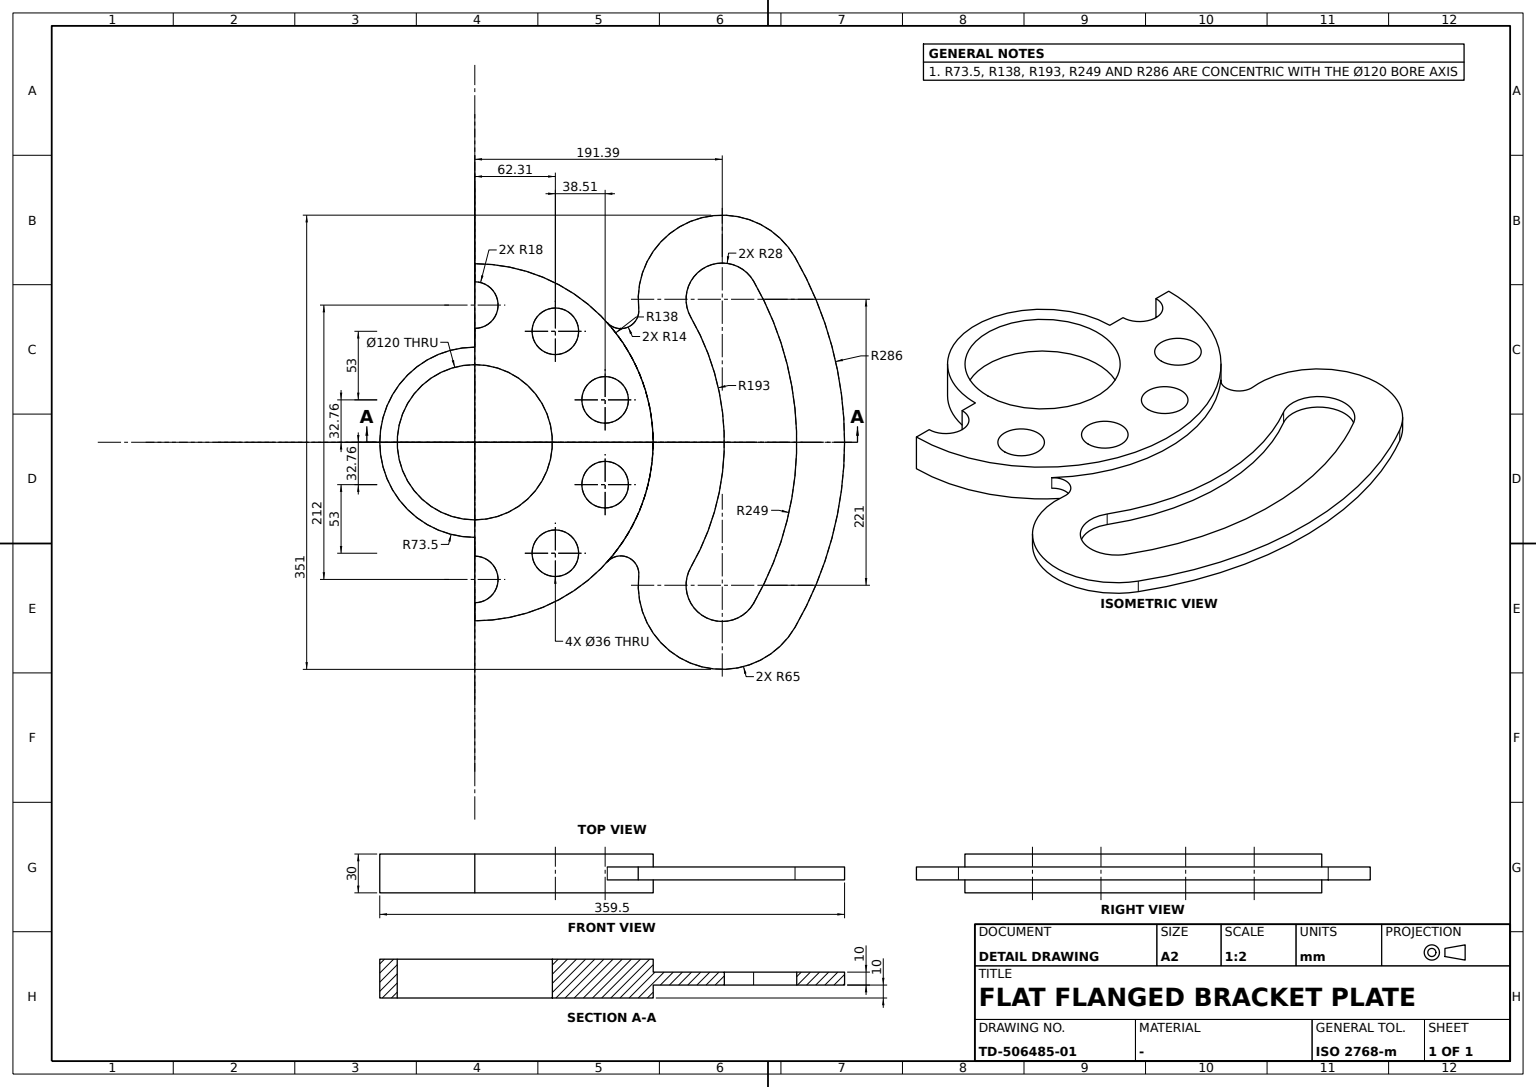
ISO-10303-21;
HEADER;
FILE_DESCRIPTION((''),'2;1');
FILE_NAME('','',(''),(''),'','','');
FILE_SCHEMA(('AUTOMOTIVE_DESIGN'));
ENDSEC;
DATA;
#1=APPLICATION_CONTEXT('');
#2=PRODUCT_CONTEXT('',#1,'mechanical');
#3=PRODUCT('','','',(#2));
#4=PRODUCT_DEFINITION_FORMATION('','',#3);
#5=PRODUCT_DEFINITION_CONTEXT('',#1,'design');
#6=PRODUCT_DEFINITION('','',#4,#5);
#7=PRODUCT_DEFINITION_SHAPE('','',#6);
#8=(LENGTH_UNIT()NAMED_UNIT(*)SI_UNIT(.MILLI.,.METRE.));
#9=(NAMED_UNIT(*)PLANE_ANGLE_UNIT()SI_UNIT($,.RADIAN.));
#10=(NAMED_UNIT(*)SI_UNIT($,.STERADIAN.)SOLID_ANGLE_UNIT());
#11=UNCERTAINTY_MEASURE_WITH_UNIT(LENGTH_MEASURE(0.005),#8,'distance_accuracy_value','');
#12=(GEOMETRIC_REPRESENTATION_CONTEXT(3)GLOBAL_UNCERTAINTY_ASSIGNED_CONTEXT((#11))GLOBAL_UNIT_ASSIGNED_CONTEXT((#8,#9,#10))REPRESENTATION_CONTEXT('',''));
#13=CARTESIAN_POINT('',(-67.7558014,62.3052367,-15.));
#14=VERTEX_POINT('',#13);
#15=CARTESIAN_POINT('',(-85.7558014,62.3052367,-15.));
#16=DIRECTION('',(0.,0.,1.));
#17=DIRECTION('',(1.,0.,0.));
#18=AXIS2_PLACEMENT_3D('',#15,#16,#17);
#19=CIRCLE('',#18,18.);
#20=EDGE_CURVE('',#14,#14,#19,.T.);
#21=ORIENTED_EDGE('',*,*,#20,.F.);
#22=EDGE_LOOP('',(#21));
#23=FACE_BOUND('',#22,.T.);
#24=CARTESIAN_POINT('',(-67.7558014,62.3052367,15.));
#25=VERTEX_POINT('',#24);
#26=CARTESIAN_POINT('',(-85.7558014,62.3052367,15.));
#27=AXIS2_PLACEMENT_3D('',#26,#16,#17);
#28=CIRCLE('',#27,18.);
#29=EDGE_CURVE('',#25,#25,#28,.T.);
#30=ORIENTED_EDGE('',*,*,#29,.T.);
#31=EDGE_LOOP('',(#30));
#32=FACE_BOUND('',#31,.T.);
#33=CARTESIAN_POINT('',(-85.7558014,62.3052367,0.));
#34=DIRECTION('',(-0.809016994,0.587785252,0.));
#35=AXIS2_PLACEMENT_3D('',#33,#16,#34);
#36=CYLINDRICAL_SURFACE('',#35,18.);
#37=ADVANCED_FACE('',(#23,#32),#36,.F.);
#38=CARTESIAN_POINT('',(96.5,167.1429029,5.));
#39=VERTEX_POINT('',#38);
#40=CARTESIAN_POINT('',(-96.5,167.1429029,5.));
#41=VERTEX_POINT('',#40);
#42=CARTESIAN_POINT('',(0.,0.,5.));
#43=AXIS2_PLACEMENT_3D('',#42,#16,#17);
#44=CIRCLE('',#43,193.);
#45=EDGE_CURVE('',#39,#41,#44,.T.);
#46=ORIENTED_EDGE('',*,*,#45,.F.);
#47=CARTESIAN_POINT('',(96.5,167.1429029,-5.));
#48=VERTEX_POINT('',#47);
#49=CARTESIAN_POINT('',(96.5,167.1429029,0.));
#50=VECTOR('',#16,1000.);
#51=LINE('',#49,#50);
#52=EDGE_CURVE('',#48,#39,#51,.T.);
#53=ORIENTED_EDGE('',*,*,#52,.F.);
#54=CARTESIAN_POINT('',(-96.5,167.1429029,-5.));
#55=VERTEX_POINT('',#54);
#56=CARTESIAN_POINT('',(0.,0.,-5.));
#57=AXIS2_PLACEMENT_3D('',#56,#16,#17);
#58=CIRCLE('',#57,193.);
#59=EDGE_CURVE('',#48,#55,#58,.T.);
#60=ORIENTED_EDGE('',*,*,#59,.T.);
#61=CARTESIAN_POINT('',(-96.5,167.1429029,0.));
#62=LINE('',#61,#50);
#63=EDGE_CURVE('',#55,#41,#62,.T.);
#64=ORIENTED_EDGE('',*,*,#63,.T.);
#65=EDGE_LOOP('',(#46,#53,#60,#64));
#66=FACE_BOUND('',#65,.T.);
#67=CARTESIAN_POINT('',(0.,0.,0.));
#68=AXIS2_PLACEMENT_3D('',#67,#16,#17);
#69=CYLINDRICAL_SURFACE('',#68,193.);
#70=ADVANCED_FACE('',(#66),#69,.T.);
#71=CARTESIAN_POINT('',(73.5,0.,-15.));
#72=VERTEX_POINT('',#71);
#73=CARTESIAN_POINT('',(88.,0.,-15.));
#74=VERTEX_POINT('',#73);
#75=CARTESIAN_POINT('',(-73.5,0.,-15.));
#76=VECTOR('',#17,1000.);
#77=LINE('',#75,#76);
#78=EDGE_CURVE('',#72,#74,#77,.T.);
#79=ORIENTED_EDGE('',*,*,#78,.T.);
#80=CARTESIAN_POINT('',(88.,0.,15.));
#81=VERTEX_POINT('',#80);
#82=LINE('',#73,#50);
#83=EDGE_CURVE('',#81,#74,#82,.F.);
#84=ORIENTED_EDGE('',*,*,#83,.F.);
#85=CARTESIAN_POINT('',(73.5,0.,15.));
#86=VERTEX_POINT('',#85);
#87=CARTESIAN_POINT('',(-73.5,0.,15.));
#88=LINE('',#87,#76);
#89=EDGE_CURVE('',#86,#81,#88,.T.);
#90=ORIENTED_EDGE('',*,*,#89,.F.);
#91=LINE('',#71,#50);
#92=EDGE_CURVE('',#72,#86,#91,.T.);
#93=ORIENTED_EDGE('',*,*,#92,.F.);
#94=EDGE_LOOP('',(#79,#84,#90,#93));
#95=FACE_BOUND('',#94,.T.);
#96=CARTESIAN_POINT('',(-73.5,0.,0.));
#97=DIRECTION('',(0.,1.,0.));
#98=DIRECTION('',(-1.,0.,0.));
#99=AXIS2_PLACEMENT_3D('',#96,#97,#98);
#100=PLANE('',#99);
#101=ADVANCED_FACE('',(#95),#100,.F.);
#102=CARTESIAN_POINT('',(-14.7558014,100.8119907,-15.));
#103=VERTEX_POINT('',#102);
#104=CARTESIAN_POINT('',(-32.7558014,100.8119907,-15.));
#105=AXIS2_PLACEMENT_3D('',#104,#16,#17);
#106=CIRCLE('',#105,18.);
#107=EDGE_CURVE('',#103,#103,#106,.T.);
#108=ORIENTED_EDGE('',*,*,#107,.F.);
#109=EDGE_LOOP('',(#108));
#110=FACE_BOUND('',#109,.T.);
#111=CARTESIAN_POINT('',(-14.7558014,100.8119907,15.));
#112=VERTEX_POINT('',#111);
#113=CARTESIAN_POINT('',(-32.7558014,100.8119907,15.));
#114=AXIS2_PLACEMENT_3D('',#113,#16,#17);
#115=CIRCLE('',#114,18.);
#116=EDGE_CURVE('',#112,#112,#115,.T.);
#117=ORIENTED_EDGE('',*,*,#116,.T.);
#118=EDGE_LOOP('',(#117));
#119=FACE_BOUND('',#118,.T.);
#120=CARTESIAN_POINT('',(-32.7558014,100.8119907,0.));
#121=DIRECTION('',(-0.309016994,0.951056516,0.));
#122=AXIS2_PLACEMENT_3D('',#120,#16,#121);
#123=CYLINDRICAL_SURFACE('',#122,18.);
#124=ADVANCED_FACE('',(#110,#119),#123,.F.);
#125=CARTESIAN_POINT('',(124.5,215.6403255,-5.));
#126=VERTEX_POINT('',#125);
#127=CARTESIAN_POINT('',(110.5,191.3916142,-5.));
#128=AXIS2_PLACEMENT_3D('',#127,#16,#17);
#129=CIRCLE('',#128,28.);
#130=EDGE_CURVE('',#48,#126,#129,.T.);
#131=ORIENTED_EDGE('',*,*,#130,.T.);
#132=CARTESIAN_POINT('',(-124.5,215.6403255,-5.));
#133=VERTEX_POINT('',#132);
#134=CIRCLE('',#57,249.);
#135=EDGE_CURVE('',#126,#133,#134,.T.);
#136=ORIENTED_EDGE('',*,*,#135,.T.);
#137=CARTESIAN_POINT('',(-110.5,191.3916142,-5.));
#138=AXIS2_PLACEMENT_3D('',#137,#16,#17);
#139=CIRCLE('',#138,28.);
#140=EDGE_CURVE('',#133,#55,#139,.T.);
#141=ORIENTED_EDGE('',*,*,#140,.T.);
#142=ORIENTED_EDGE('',*,*,#59,.F.);
#143=EDGE_LOOP('',(#131,#136,#141,#142));
#144=FACE_BOUND('',#143,.T.);
#145=CARTESIAN_POINT('',(-92.4269535,102.4756472,-5.));
#146=VERTEX_POINT('',#145);
#147=CARTESIAN_POINT('',(-103.344735,126.786644,-5.));
#148=VERTEX_POINT('',#147);
#149=CARTESIAN_POINT('',(-101.803601,112.8717273,-5.));
#150=AXIS2_PLACEMENT_3D('',#149,#16,#17);
#151=CIRCLE('',#150,14.);
#152=EDGE_CURVE('',#146,#148,#151,.T.);
#153=ORIENTED_EDGE('',*,*,#152,.T.);
#154=CARTESIAN_POINT('',(-143.,247.6832655,-5.));
#155=VERTEX_POINT('',#154);
#156=CIRCLE('',#138,65.);
#157=EDGE_CURVE('',#155,#148,#156,.T.);
#158=ORIENTED_EDGE('',*,*,#157,.F.);
#159=CARTESIAN_POINT('',(143.,247.6832655,-5.));
#160=VERTEX_POINT('',#159);
#161=CIRCLE('',#57,286.);
#162=EDGE_CURVE('',#160,#155,#161,.T.);
#163=ORIENTED_EDGE('',*,*,#162,.F.);
#164=CARTESIAN_POINT('',(103.344735,126.786644,-5.));
#165=VERTEX_POINT('',#164);
#166=CIRCLE('',#128,65.);
#167=EDGE_CURVE('',#165,#160,#166,.T.);
#168=ORIENTED_EDGE('',*,*,#167,.F.);
#169=CARTESIAN_POINT('',(92.4269535,102.4756472,-5.));
#170=VERTEX_POINT('',#169);
#171=CARTESIAN_POINT('',(101.803601,112.8717273,-5.));
#172=AXIS2_PLACEMENT_3D('',#171,#16,#17);
#173=CIRCLE('',#172,14.);
#174=EDGE_CURVE('',#165,#170,#173,.T.);
#175=ORIENTED_EDGE('',*,*,#174,.T.);
#176=CIRCLE('',#57,138.);
#177=EDGE_CURVE('',#170,#146,#176,.T.);
#178=ORIENTED_EDGE('',*,*,#177,.T.);
#179=EDGE_LOOP('',(#153,#158,#163,#168,#175,#178));
#180=FACE_BOUND('',#179,.T.);
#181=PLANE('',#57);
#182=ADVANCED_FACE('',(#144,#180),#181,.F.);
#183=CARTESIAN_POINT('',(60.,0.,15.));
#184=VERTEX_POINT('',#183);
#185=CARTESIAN_POINT('',(0.,0.,15.));
#186=AXIS2_PLACEMENT_3D('',#185,#16,#17);
#187=CIRCLE('',#186,60.);
#188=EDGE_CURVE('',#184,#184,#187,.T.);
#189=ORIENTED_EDGE('',*,*,#188,.T.);
#190=EDGE_LOOP('',(#189));
#191=FACE_BOUND('',#190,.T.);
#192=CARTESIAN_POINT('',(60.,0.,-15.));
#193=VERTEX_POINT('',#192);
#194=CARTESIAN_POINT('',(0.,0.,-15.));
#195=AXIS2_PLACEMENT_3D('',#194,#16,#17);
#196=CIRCLE('',#195,60.);
#197=EDGE_CURVE('',#193,#193,#196,.T.);
#198=ORIENTED_EDGE('',*,*,#197,.F.);
#199=EDGE_LOOP('',(#198));
#200=FACE_BOUND('',#199,.T.);
#201=CYLINDRICAL_SURFACE('',#68,60.);
#202=ADVANCED_FACE('',(#191,#200),#201,.F.);
#203=CARTESIAN_POINT('',(103.7558014,62.3052367,15.));
#204=VERTEX_POINT('',#203);
#205=CARTESIAN_POINT('',(85.7558014,62.3052367,15.));
#206=AXIS2_PLACEMENT_3D('',#205,#16,#17);
#207=CIRCLE('',#206,18.);
#208=EDGE_CURVE('',#204,#204,#207,.T.);
#209=ORIENTED_EDGE('',*,*,#208,.T.);
#210=EDGE_LOOP('',(#209));
#211=FACE_BOUND('',#210,.T.);
#212=CARTESIAN_POINT('',(103.7558014,62.3052367,-15.));
#213=VERTEX_POINT('',#212);
#214=CARTESIAN_POINT('',(85.7558014,62.3052367,-15.));
#215=AXIS2_PLACEMENT_3D('',#214,#16,#17);
#216=CIRCLE('',#215,18.);
#217=EDGE_CURVE('',#213,#213,#216,.T.);
#218=ORIENTED_EDGE('',*,*,#217,.F.);
#219=EDGE_LOOP('',(#218));
#220=FACE_BOUND('',#219,.T.);
#221=CARTESIAN_POINT('',(85.7558014,62.3052367,0.));
#222=DIRECTION('',(0.809016994,0.587785252,0.));
#223=AXIS2_PLACEMENT_3D('',#221,#16,#222);
#224=CYLINDRICAL_SURFACE('',#223,18.);
#225=ADVANCED_FACE('',(#211,#220),#224,.F.);
#226=CARTESIAN_POINT('',(-88.,0.,15.));
#227=VERTEX_POINT('',#226);
#228=CARTESIAN_POINT('',(-124.,0.,15.));
#229=VERTEX_POINT('',#228);
#230=CARTESIAN_POINT('',(-106.,0.,15.));
#231=AXIS2_PLACEMENT_3D('',#230,#16,#17);
#232=CIRCLE('',#231,18.);
#233=EDGE_CURVE('',#227,#229,#232,.T.);
#234=ORIENTED_EDGE('',*,*,#233,.T.);
#235=CARTESIAN_POINT('',(-124.,0.,-15.));
#236=VERTEX_POINT('',#235);
#237=LINE('',#235,#50);
#238=EDGE_CURVE('',#236,#229,#237,.T.);
#239=ORIENTED_EDGE('',*,*,#238,.F.);
#240=CARTESIAN_POINT('',(-88.,0.,-15.));
#241=VERTEX_POINT('',#240);
#242=CARTESIAN_POINT('',(-106.,0.,-15.));
#243=AXIS2_PLACEMENT_3D('',#242,#16,#17);
#244=CIRCLE('',#243,18.);
#245=EDGE_CURVE('',#241,#236,#244,.T.);
#246=ORIENTED_EDGE('',*,*,#245,.F.);
#247=LINE('',#240,#50);
#248=EDGE_CURVE('',#227,#241,#247,.F.);
#249=ORIENTED_EDGE('',*,*,#248,.F.);
#250=EDGE_LOOP('',(#234,#239,#246,#249));
#251=FACE_BOUND('',#250,.T.);
#252=CARTESIAN_POINT('',(-106.,0.,0.));
#253=AXIS2_PLACEMENT_3D('',#252,#16,#98);
#254=CYLINDRICAL_SURFACE('',#253,18.);
#255=ADVANCED_FACE('',(#251),#254,.F.);
#256=CARTESIAN_POINT('',(138.,0.,-15.));
#257=VERTEX_POINT('',#256);
#258=CARTESIAN_POINT('',(138.,0.,15.));
#259=VERTEX_POINT('',#258);
#260=LINE('',#256,#50);
#261=EDGE_CURVE('',#257,#259,#260,.T.);
#262=ORIENTED_EDGE('',*,*,#261,.F.);
#263=CARTESIAN_POINT('',(-138.,0.,-15.));
#264=VERTEX_POINT('',#263);
#265=CIRCLE('',#195,138.);
#266=EDGE_CURVE('',#257,#264,#265,.T.);
#267=ORIENTED_EDGE('',*,*,#266,.T.);
#268=CARTESIAN_POINT('',(-138.,0.,15.));
#269=VERTEX_POINT('',#268);
#270=LINE('',#263,#50);
#271=EDGE_CURVE('',#264,#269,#270,.T.);
#272=ORIENTED_EDGE('',*,*,#271,.T.);
#273=CIRCLE('',#186,138.);
#274=EDGE_CURVE('',#259,#269,#273,.T.);
#275=ORIENTED_EDGE('',*,*,#274,.F.);
#276=EDGE_LOOP('',(#262,#267,#272,#275));
#277=FACE_BOUND('',#276,.T.);
#278=ORIENTED_EDGE('',*,*,#177,.F.);
#279=CARTESIAN_POINT('',(92.4269535,102.4756472,5.));
#280=VERTEX_POINT('',#279);
#281=CARTESIAN_POINT('',(92.4269535,102.4756472,0.));
#282=LINE('',#281,#50);
#283=EDGE_CURVE('',#170,#280,#282,.T.);
#284=ORIENTED_EDGE('',*,*,#283,.T.);
#285=CARTESIAN_POINT('',(-92.4269535,102.4756472,5.));
#286=VERTEX_POINT('',#285);
#287=CIRCLE('',#43,138.);
#288=EDGE_CURVE('',#280,#286,#287,.T.);
#289=ORIENTED_EDGE('',*,*,#288,.T.);
#290=CARTESIAN_POINT('',(-92.4269535,102.4756472,0.));
#291=LINE('',#290,#50);
#292=EDGE_CURVE('',#146,#286,#291,.T.);
#293=ORIENTED_EDGE('',*,*,#292,.F.);
#294=EDGE_LOOP('',(#278,#284,#289,#293));
#295=FACE_BOUND('',#294,.T.);
#296=CYLINDRICAL_SURFACE('',#68,138.);
#297=ADVANCED_FACE('',(#277,#295),#296,.T.);
#298=ORIENTED_EDGE('',*,*,#63,.F.);
#299=ORIENTED_EDGE('',*,*,#140,.F.);
#300=CARTESIAN_POINT('',(-124.5,215.6403255,5.));
#301=VERTEX_POINT('',#300);
#302=CARTESIAN_POINT('',(-124.5,215.6403255,0.));
#303=LINE('',#302,#50);
#304=EDGE_CURVE('',#133,#301,#303,.T.);
#305=ORIENTED_EDGE('',*,*,#304,.T.);
#306=CARTESIAN_POINT('',(-110.5,191.3916142,5.));
#307=AXIS2_PLACEMENT_3D('',#306,#16,#17);
#308=CIRCLE('',#307,28.);
#309=EDGE_CURVE('',#301,#41,#308,.T.);
#310=ORIENTED_EDGE('',*,*,#309,.T.);
#311=EDGE_LOOP('',(#298,#299,#305,#310));
#312=FACE_BOUND('',#311,.T.);
#313=CARTESIAN_POINT('',(-110.5,191.3916142,0.));
#314=AXIS2_PLACEMENT_3D('',#313,#16,#17);
#315=CYLINDRICAL_SURFACE('',#314,28.);
#316=ADVANCED_FACE('',(#312),#315,.F.);
#317=ORIENTED_EDGE('',*,*,#238,.T.);
#318=EDGE_CURVE('',#269,#229,#88,.T.);
#319=ORIENTED_EDGE('',*,*,#318,.F.);
#320=ORIENTED_EDGE('',*,*,#271,.F.);
#321=EDGE_CURVE('',#264,#236,#77,.T.);
#322=ORIENTED_EDGE('',*,*,#321,.T.);
#323=EDGE_LOOP('',(#317,#319,#320,#322));
#324=FACE_BOUND('',#323,.T.);
#325=ADVANCED_FACE('',(#324),#100,.F.);
#326=CARTESIAN_POINT('',(50.7558014,100.8119907,-15.));
#327=VERTEX_POINT('',#326);
#328=CARTESIAN_POINT('',(32.7558014,100.8119907,-15.));
#329=AXIS2_PLACEMENT_3D('',#328,#16,#17);
#330=CIRCLE('',#329,18.);
#331=EDGE_CURVE('',#327,#327,#330,.T.);
#332=ORIENTED_EDGE('',*,*,#331,.F.);
#333=EDGE_LOOP('',(#332));
#334=FACE_BOUND('',#333,.T.);
#335=CARTESIAN_POINT('',(50.7558014,100.8119907,15.));
#336=VERTEX_POINT('',#335);
#337=CARTESIAN_POINT('',(32.7558014,100.8119907,15.));
#338=AXIS2_PLACEMENT_3D('',#337,#16,#17);
#339=CIRCLE('',#338,18.);
#340=EDGE_CURVE('',#336,#336,#339,.T.);
#341=ORIENTED_EDGE('',*,*,#340,.T.);
#342=EDGE_LOOP('',(#341));
#343=FACE_BOUND('',#342,.T.);
#344=CARTESIAN_POINT('',(32.7558014,100.8119907,0.));
#345=DIRECTION('',(0.309016994,0.951056516,0.));
#346=AXIS2_PLACEMENT_3D('',#344,#16,#345);
#347=CYLINDRICAL_SURFACE('',#346,18.);
#348=ADVANCED_FACE('',(#334,#343),#347,.F.);
#349=ORIENTED_EDGE('',*,*,#340,.F.);
#350=EDGE_LOOP('',(#349));
#351=FACE_BOUND('',#350,.T.);
#352=CARTESIAN_POINT('',(124.,0.,15.));
#353=VERTEX_POINT('',#352);
#354=CARTESIAN_POINT('',(106.,0.,15.));
#355=AXIS2_PLACEMENT_3D('',#354,#16,#17);
#356=CIRCLE('',#355,18.);
#357=EDGE_CURVE('',#353,#81,#356,.T.);
#358=ORIENTED_EDGE('',*,*,#357,.F.);
#359=EDGE_CURVE('',#353,#259,#88,.T.);
#360=ORIENTED_EDGE('',*,*,#359,.T.);
#361=ORIENTED_EDGE('',*,*,#274,.T.);
#362=ORIENTED_EDGE('',*,*,#318,.T.);
#363=ORIENTED_EDGE('',*,*,#233,.F.);
#364=VERTEX_POINT('',#87);
#365=EDGE_CURVE('',#227,#364,#88,.T.);
#366=ORIENTED_EDGE('',*,*,#365,.T.);
#367=CIRCLE('',#186,73.5);
#368=EDGE_CURVE('',#364,#86,#367,.T.);
#369=ORIENTED_EDGE('',*,*,#368,.T.);
#370=ORIENTED_EDGE('',*,*,#89,.T.);
#371=EDGE_LOOP('',(#358,#360,#361,#362,#363,#366,#369,#370));
#372=FACE_BOUND('',#371,.T.);
#373=ORIENTED_EDGE('',*,*,#188,.F.);
#374=EDGE_LOOP('',(#373));
#375=FACE_BOUND('',#374,.T.);
#376=ORIENTED_EDGE('',*,*,#208,.F.);
#377=EDGE_LOOP('',(#376));
#378=FACE_BOUND('',#377,.T.);
#379=ORIENTED_EDGE('',*,*,#116,.F.);
#380=EDGE_LOOP('',(#379));
#381=FACE_BOUND('',#380,.T.);
#382=ORIENTED_EDGE('',*,*,#29,.F.);
#383=EDGE_LOOP('',(#382));
#384=FACE_BOUND('',#383,.T.);
#385=PLANE('',#186);
#386=ADVANCED_FACE('',(#351,#372,#375,#378,#381,#384),#385,.T.);
#387=CARTESIAN_POINT('',(103.344735,126.786644,5.));
#388=VERTEX_POINT('',#387);
#389=CARTESIAN_POINT('',(101.803601,112.8717273,5.));
#390=AXIS2_PLACEMENT_3D('',#389,#16,#17);
#391=CIRCLE('',#390,14.);
#392=EDGE_CURVE('',#388,#280,#391,.T.);
#393=ORIENTED_EDGE('',*,*,#392,.T.);
#394=ORIENTED_EDGE('',*,*,#283,.F.);
#395=ORIENTED_EDGE('',*,*,#174,.F.);
#396=CARTESIAN_POINT('',(103.344735,126.786644,0.));
#397=LINE('',#396,#50);
#398=EDGE_CURVE('',#165,#388,#397,.T.);
#399=ORIENTED_EDGE('',*,*,#398,.T.);
#400=EDGE_LOOP('',(#393,#394,#395,#399));
#401=FACE_BOUND('',#400,.T.);
#402=CARTESIAN_POINT('',(101.803601,112.8717273,0.));
#403=AXIS2_PLACEMENT_3D('',#402,#16,#17);
#404=CYLINDRICAL_SURFACE('',#403,14.);
#405=ADVANCED_FACE('',(#401),#404,.F.);
#406=CARTESIAN_POINT('',(-103.344735,126.786644,5.));
#407=VERTEX_POINT('',#406);
#408=CARTESIAN_POINT('',(-101.803601,112.8717273,5.));
#409=AXIS2_PLACEMENT_3D('',#408,#16,#17);
#410=CIRCLE('',#409,14.);
#411=EDGE_CURVE('',#286,#407,#410,.T.);
#412=ORIENTED_EDGE('',*,*,#411,.T.);
#413=CARTESIAN_POINT('',(-103.344735,126.786644,0.));
#414=LINE('',#413,#50);
#415=EDGE_CURVE('',#148,#407,#414,.T.);
#416=ORIENTED_EDGE('',*,*,#415,.F.);
#417=ORIENTED_EDGE('',*,*,#152,.F.);
#418=ORIENTED_EDGE('',*,*,#292,.T.);
#419=EDGE_LOOP('',(#412,#416,#417,#418));
#420=FACE_BOUND('',#419,.T.);
#421=CARTESIAN_POINT('',(-101.803601,112.8717273,0.));
#422=AXIS2_PLACEMENT_3D('',#421,#16,#17);
#423=CYLINDRICAL_SURFACE('',#422,14.);
#424=ADVANCED_FACE('',(#420),#423,.F.);
#425=ORIENTED_EDGE('',*,*,#107,.T.);
#426=EDGE_LOOP('',(#425));
#427=FACE_BOUND('',#426,.T.);
#428=ORIENTED_EDGE('',*,*,#331,.T.);
#429=EDGE_LOOP('',(#428));
#430=FACE_BOUND('',#429,.T.);
#431=ORIENTED_EDGE('',*,*,#217,.T.);
#432=EDGE_LOOP('',(#431));
#433=FACE_BOUND('',#432,.T.);
#434=CARTESIAN_POINT('',(124.,0.,-15.));
#435=VERTEX_POINT('',#434);
#436=CARTESIAN_POINT('',(106.,0.,-15.));
#437=AXIS2_PLACEMENT_3D('',#436,#16,#17);
#438=CIRCLE('',#437,18.);
#439=EDGE_CURVE('',#435,#74,#438,.T.);
#440=ORIENTED_EDGE('',*,*,#439,.T.);
#441=ORIENTED_EDGE('',*,*,#78,.F.);
#442=VERTEX_POINT('',#75);
#443=CIRCLE('',#195,73.5);
#444=EDGE_CURVE('',#442,#72,#443,.T.);
#445=ORIENTED_EDGE('',*,*,#444,.F.);
#446=EDGE_CURVE('',#241,#442,#77,.T.);
#447=ORIENTED_EDGE('',*,*,#446,.F.);
#448=ORIENTED_EDGE('',*,*,#245,.T.);
#449=ORIENTED_EDGE('',*,*,#321,.F.);
#450=ORIENTED_EDGE('',*,*,#266,.F.);
#451=EDGE_CURVE('',#435,#257,#77,.T.);
#452=ORIENTED_EDGE('',*,*,#451,.F.);
#453=EDGE_LOOP('',(#440,#441,#445,#447,#448,#449,#450,#452));
#454=FACE_BOUND('',#453,.T.);
#455=ORIENTED_EDGE('',*,*,#20,.T.);
#456=EDGE_LOOP('',(#455));
#457=FACE_BOUND('',#456,.T.);
#458=ORIENTED_EDGE('',*,*,#197,.T.);
#459=EDGE_LOOP('',(#458));
#460=FACE_BOUND('',#459,.T.);
#461=PLANE('',#195);
#462=ADVANCED_FACE('',(#427,#430,#433,#454,#457,#460),#461,.F.);
#463=CARTESIAN_POINT('',(-143.,247.6832655,5.));
#464=VERTEX_POINT('',#463);
#465=CIRCLE('',#307,65.);
#466=EDGE_CURVE('',#464,#407,#465,.T.);
#467=ORIENTED_EDGE('',*,*,#466,.F.);
#468=CARTESIAN_POINT('',(-143.,247.6832655,0.));
#469=LINE('',#468,#50);
#470=EDGE_CURVE('',#155,#464,#469,.T.);
#471=ORIENTED_EDGE('',*,*,#470,.F.);
#472=ORIENTED_EDGE('',*,*,#157,.T.);
#473=ORIENTED_EDGE('',*,*,#415,.T.);
#474=EDGE_LOOP('',(#467,#471,#472,#473));
#475=FACE_BOUND('',#474,.T.);
#476=CYLINDRICAL_SURFACE('',#314,65.);
#477=ADVANCED_FACE('',(#475),#476,.T.);
#478=CARTESIAN_POINT('',(143.,247.6832655,5.));
#479=VERTEX_POINT('',#478);
#480=CIRCLE('',#43,286.);
#481=EDGE_CURVE('',#479,#464,#480,.T.);
#482=ORIENTED_EDGE('',*,*,#481,.F.);
#483=CARTESIAN_POINT('',(143.,247.6832655,0.));
#484=LINE('',#483,#50);
#485=EDGE_CURVE('',#160,#479,#484,.T.);
#486=ORIENTED_EDGE('',*,*,#485,.F.);
#487=ORIENTED_EDGE('',*,*,#162,.T.);
#488=ORIENTED_EDGE('',*,*,#470,.T.);
#489=EDGE_LOOP('',(#482,#486,#487,#488));
#490=FACE_BOUND('',#489,.T.);
#491=CYLINDRICAL_SURFACE('',#68,286.);
#492=ADVANCED_FACE('',(#490),#491,.T.);
#493=ORIENTED_EDGE('',*,*,#446,.T.);
#494=LINE('',#75,#50);
#495=EDGE_CURVE('',#442,#364,#494,.T.);
#496=ORIENTED_EDGE('',*,*,#495,.T.);
#497=ORIENTED_EDGE('',*,*,#365,.F.);
#498=ORIENTED_EDGE('',*,*,#248,.T.);
#499=EDGE_LOOP('',(#493,#496,#497,#498));
#500=FACE_BOUND('',#499,.T.);
#501=ADVANCED_FACE('',(#500),#100,.F.);
#502=ORIENTED_EDGE('',*,*,#167,.T.);
#503=ORIENTED_EDGE('',*,*,#485,.T.);
#504=CARTESIAN_POINT('',(110.5,191.3916142,5.));
#505=AXIS2_PLACEMENT_3D('',#504,#16,#17);
#506=CIRCLE('',#505,65.);
#507=EDGE_CURVE('',#388,#479,#506,.T.);
#508=ORIENTED_EDGE('',*,*,#507,.F.);
#509=ORIENTED_EDGE('',*,*,#398,.F.);
#510=EDGE_LOOP('',(#502,#503,#508,#509));
#511=FACE_BOUND('',#510,.T.);
#512=CARTESIAN_POINT('',(110.5,191.3916142,0.));
#513=AXIS2_PLACEMENT_3D('',#512,#16,#17);
#514=CYLINDRICAL_SURFACE('',#513,65.);
#515=ADVANCED_FACE('',(#511),#514,.T.);
#516=CARTESIAN_POINT('',(124.5,215.6403255,5.));
#517=VERTEX_POINT('',#516);
#518=CARTESIAN_POINT('',(124.5,215.6403255,0.));
#519=LINE('',#518,#50);
#520=EDGE_CURVE('',#126,#517,#519,.T.);
#521=ORIENTED_EDGE('',*,*,#520,.F.);
#522=ORIENTED_EDGE('',*,*,#130,.F.);
#523=ORIENTED_EDGE('',*,*,#52,.T.);
#524=CIRCLE('',#505,28.);
#525=EDGE_CURVE('',#39,#517,#524,.T.);
#526=ORIENTED_EDGE('',*,*,#525,.T.);
#527=EDGE_LOOP('',(#521,#522,#523,#526));
#528=FACE_BOUND('',#527,.T.);
#529=CYLINDRICAL_SURFACE('',#513,28.);
#530=ADVANCED_FACE('',(#528),#529,.F.);
#531=ORIENTED_EDGE('',*,*,#135,.F.);
#532=ORIENTED_EDGE('',*,*,#520,.T.);
#533=CIRCLE('',#43,249.);
#534=EDGE_CURVE('',#517,#301,#533,.T.);
#535=ORIENTED_EDGE('',*,*,#534,.T.);
#536=ORIENTED_EDGE('',*,*,#304,.F.);
#537=EDGE_LOOP('',(#531,#532,#535,#536));
#538=FACE_BOUND('',#537,.T.);
#539=CYLINDRICAL_SURFACE('',#68,249.);
#540=ADVANCED_FACE('',(#538),#539,.F.);
#541=ORIENTED_EDGE('',*,*,#534,.F.);
#542=ORIENTED_EDGE('',*,*,#525,.F.);
#543=ORIENTED_EDGE('',*,*,#45,.T.);
#544=ORIENTED_EDGE('',*,*,#309,.F.);
#545=EDGE_LOOP('',(#541,#542,#543,#544));
#546=FACE_BOUND('',#545,.T.);
#547=ORIENTED_EDGE('',*,*,#507,.T.);
#548=ORIENTED_EDGE('',*,*,#481,.T.);
#549=ORIENTED_EDGE('',*,*,#466,.T.);
#550=ORIENTED_EDGE('',*,*,#411,.F.);
#551=ORIENTED_EDGE('',*,*,#288,.F.);
#552=ORIENTED_EDGE('',*,*,#392,.F.);
#553=EDGE_LOOP('',(#547,#548,#549,#550,#551,#552));
#554=FACE_BOUND('',#553,.T.);
#555=PLANE('',#43);
#556=ADVANCED_FACE('',(#546,#554),#555,.T.);
#557=ORIENTED_EDGE('',*,*,#444,.T.);
#558=ORIENTED_EDGE('',*,*,#92,.T.);
#559=ORIENTED_EDGE('',*,*,#368,.F.);
#560=ORIENTED_EDGE('',*,*,#495,.F.);
#561=EDGE_LOOP('',(#557,#558,#559,#560));
#562=FACE_BOUND('',#561,.T.);
#563=CYLINDRICAL_SURFACE('',#68,73.5);
#564=ADVANCED_FACE('',(#562),#563,.T.);
#565=ORIENTED_EDGE('',*,*,#357,.T.);
#566=ORIENTED_EDGE('',*,*,#83,.T.);
#567=ORIENTED_EDGE('',*,*,#439,.F.);
#568=LINE('',#434,#50);
#569=EDGE_CURVE('',#435,#353,#568,.T.);
#570=ORIENTED_EDGE('',*,*,#569,.T.);
#571=EDGE_LOOP('',(#565,#566,#567,#570));
#572=FACE_BOUND('',#571,.T.);
#573=CARTESIAN_POINT('',(106.,0.,0.));
#574=AXIS2_PLACEMENT_3D('',#573,#16,#17);
#575=CYLINDRICAL_SURFACE('',#574,18.);
#576=ADVANCED_FACE('',(#572),#575,.F.);
#577=ORIENTED_EDGE('',*,*,#569,.F.);
#578=ORIENTED_EDGE('',*,*,#451,.T.);
#579=ORIENTED_EDGE('',*,*,#261,.T.);
#580=ORIENTED_EDGE('',*,*,#359,.F.);
#581=EDGE_LOOP('',(#577,#578,#579,#580));
#582=FACE_BOUND('',#581,.T.);
#583=ADVANCED_FACE('',(#582),#100,.F.);
#584=CLOSED_SHELL('',(#37,#70,#101,#124,#182,#202,#225,#255,#297,#316,#325,#348,#386,#405,#424,#462,#477,#492,#501,#515,#530,#540,#556,#564,#576,#583));
#585=MANIFOLD_SOLID_BREP('',#584);
#586=ADVANCED_BREP_SHAPE_REPRESENTATION('',(#585),#12);
#587=SHAPE_DEFINITION_REPRESENTATION(#7,#586);
ENDSEC;
END-ISO-10303-21;
